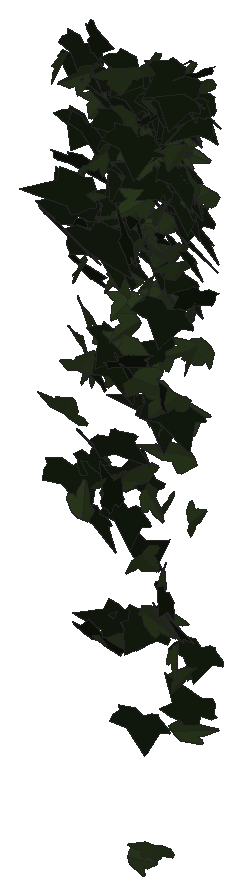
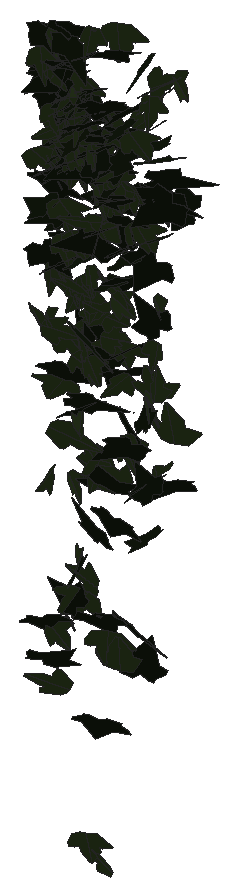
# SketchUp Ruby script. Lengths in millimetres.
U = 1.mm
M = Sketchup.active_model
def pt(a) = Geom::Point3d.new(a.map { |v| v * U })
def face(e, loops, mat)
  f = e.add_face(loops[0].map { |a| pt(a) })
  loops[1..].each { |l| e.add_face(l.map { |a| pt(a) }).erase! }
  f.material = f.back_material = mat if mat
  f
end
# faces: each face lists its corners as indices into pts; further lists are holes
def faces(e, pts, list, mat = nil) = list.each { |f| face(e, (f[0].is_a?(Array) ? f : [f]).map { |l| l.map { |i| pts[i] } }, mat) }
# xy, xz, yz: faces in a plane at the given z, y or x. An outline is a flat list of corners, or four numbers for a rectangle; further outlines are holes
def ring(l) = l.size == 4 ? [[l[0], l[1]], [l[2], l[1]], [l[2], l[3]], [l[0], l[3]]] : l.each_slice(2).to_a
def flat(e, list, mat, &to3) = list.each { |f| face(e, (f[0].is_a?(Array) ? f : [f]).map { |l| ring(l).map { |u, v| to3.(u, v) } }, mat) }
def xy(e, z, list, mat = nil) = flat(e, list, mat) { |x, y| [x, y, z] }
def xz(e, y, list, mat = nil) = flat(e, list, mat) { |x, z| [x, y, z] }
def yz(e, x, list, mat = nil) = flat(e, list, mat) { |y, z| [x, y, z] }
def lines(e, pts, list) = list.each { |a, b| e.add_line(pt(pts[a]), pt(pts[b])) }
# prism: a flat outline (further loops are holes) pulled along v
def prism(e, loops, v, mat = nil)
  f = face(e, loops, mat); d = Geom::Vector3d.new(v.map { |x| x * U })
  f.pushpull(f.normal.samedirection?(d) ? d.length : -d.length)
end
def box(e, o, s, mat = nil) = prism(e, [[o, [o[0] + s[0], o[1], o[2]], [o[0] + s[0], o[1] + s[1], o[2]], [o[0], o[1] + s[1], o[2]]]], [0, 0, s[2]], mat)
def at(x, y, z, deg = 0) = Geom::Transformation.translation(pt([x, y, z])) * Geom::Transformation.rotation(ORIGIN, Z_AXIS, deg.degrees)
def axes(o, x, y, z) = Geom::Transformation.new([*x, 0, *y, 0, *z, 0, *pt(o).to_a, 1])
def part(name) = M.definitions.add(name)
# library, detail: a bought-in or finely detailed component or shape, given as its bounding box
def library(name, o, s) = part(name).tap { |d| box(d.entities, o, s) }
def detail(e, o, s) = box(e.add_group.entities, o, s)
def put(e, d, t, mat = nil) = e.add_instance(d, t).tap { |i| i.material = mat if mat }
def group(e, t, mat = nil) = e.add_group.tap { |g| g.transformation = t; g.material = mat if mat }.entities
root = M.entities
M.materials.add("efeu1").color = [18, 25, 13]
M.materials.add("efeu2").color = [43, 57, 29]
c1 = part("ivyleaf_10")
p = [[0,12.8,-0.8],[-1.5,51.3,-10.9],[-4.9,51,-11.6],[-13.6,26.5,-7.3],[-13.2,15.9,-4.6],[-21.1,19.3,-7.2],
  [-29.5,16.3,-8.3],[-29.2,8.3,-6.2],[-19.7,-9.8,0.5],[-7.6,-13,4],[1,-12.2,5.8],[-0.4,51.1,-11.1],
  [-1.5,51.1,-10.9],[1,-12.4,5.9],[16.9,-12.4,3.5],[35.1,9.1,-5.1],[35,12.9,-6.1],[20.5,16.4,-4.9],
  [15.8,15,-3.8],[15.3,27.6,-7.1],[12.8,31.3,-7.8]]
faces(c1.entities,p,[[0,1,2,3,4,5,6,7,8,9,10],[11,12,0,13,14,15,16,17,18,19,20]],"efeu2")
c2 = part("ivyleaf_9")
p = [[39.1,54.8,31.7],[34.5,51.8,30.2],[-5.3,25.2,17.3],[-17.9,28.3,20.9],[-21.6,21.7,17],[-20.2,4.3,5.3],
  [-22.9,-0.3,2.5],[-17.1,-4,-0.6],[-2,-2.1,-1.2],[-0.7,-15.4,-10.1],[16.6,-22.3,-16.7],[21.1,-15.1,-12.5],
  [32.7,-10.7,-11],[46.1,-1.8,-6.6],[30.8,11.2,3.8]]
faces(c2.entities,p,[[0,1,2,3,4,5,6,7,8,9,10,11,12,13,14]],"efeu1")
put(root,c1,axes([1159.9,911.5,1594.2],[0.32513,-0.7471,0.35],[0.24171,-0.32935,-0.76501],[1.55146,0.20788,0.04584]))
put(root,c1,axes([1156.6,970.6,1037.6],[-1.07605,0.47625,0.41907],[0.55178,-0.30531,0.73812],[1.07388,0.63409,0.04065]))
put(root,c2,axes([1144.9,952.8,1391],[1.62557,0.19363,0.00813],[0.01368,0.00506,-0.87579],[-0.36858,0.85415,0.00335]))
put(root,c1,axes([1164.6,958.1,1198.9],[0.31371,-0.73635,0.01947],[-0.00898,-0.021,-0.75452],[1.40188,0.16464,-0.00919]))
put(root,c1,axes([1169.3,960.4,1115.8],[-0.99769,0.51043,0.28692],[-0.38193,0.20516,-0.73164],[-1.04692,-0.56128,-0.00651]))
put(root,c1,axes([1175.6,969.8,991.9],[0.31863,-0.24231,0.79637],[-0.89433,0.643,0.29443],[-1.30769,-0.49879,-0.00731]))
put(root,c1,axes([1157.6,923.9,940.9],[-1.65035,0.0751,0.31552],[0.57406,-0.14434,0.86332],[0.22691,0.91141,0.11072]))
put(root,c2,axes([1143,984.8,1174.3],[1.23837,-0.18816,-0.40424],[0.76944,-0.05265,0.67526],[-0.35791,-0.76421,0.05301]))
put(root,c2,axes([1165.8,964.2,1278.3],[0.99581,0.56044,0.06902],[0.09755,0.04657,-0.7667],[-1.07026,0.5257,-0.00566]))
put(root,c2,axes([1166.9,994.2,986.3],[-0.32289,-0.14497,0.77042],[-0.11432,-0.78354,-0.16066],[1.48761,-0.09168,0.15487]))
put(root,c2,axes([1159,939.7,1587.2],[0.69414,-0.6805,-0.43662],[-0.30896,0.4076,-0.77087],[1.50744,0.39689,0.04306]))
put(root,c1,axes([1175.9,966,1015.5],[0.64827,-0.72726,-0.00598],[-0.0036,0.00572,-0.80307],[1.38416,0.34063,0.00072]))
put(root,c2,axes([1166.5,960.3,1600.1],[-0.28503,-0.77891,0.2669],[-0.06559,-0.26512,-0.79303],[1.56566,-0.15291,0.01537]))
put(root,c2,axes([1160.8,983,1536.1],[0.378,-0.7746,-0.18675],[-0.07957,0.18207,-0.79965],[1.51437,0.20291,0.0046]))
put(root,c2,axes([1174.5,957.7,1459.9],[-0.82889,-0.61017,0.31763],[0.07587,-0.39769,-0.70932],[1.30699,-0.36388,0.24261]))
put(root,c1,axes([1178,942.1,1377],[0.47899,-0.80206,0.1969],[0.08656,-0.19207,-0.8405],[1.56941,0.25538,-0.01374]))
put(root,c2,axes([1158.5,982.7,860.2],[1.07212,-0.24968,-0.50922],[0.88478,-0.20781,0.61618],[-0.61825,-0.73038,-0.00124]))
put(root,c2,axes([1174.8,975.2,1316.8],[-0.47432,-0.68277,0.30544],[0.08624,-0.33514,-0.71219],[1.42094,-0.20758,0.14519]))
put(root,c1,axes([1186.8,950.5,1562.9],[-0.32026,-0.75005,-0.31521],[0.13106,0.3076,-0.76869],[1.54287,-0.18182,-0.00013]))
put(root,c1,axes([1180.6,940,1021.9],[-1.07087,-0.52934,0.14175],[0.19473,0.09812,0.77253],[-1.0246,0.57189,-0.00134]))
put(root,c2,axes([1175.3,921.5,845.1],[-0.49527,-0.77132,-0.42107],[0.33043,0.38536,-0.81321],[1.6395,-0.31067,0.0367]))
put(root,c1,axes([1196.5,981,1505.4],[-0.74088,-0.61442,0.38107],[-0.16276,-0.39063,-0.71719],[1.36636,-0.37969,0.1212]))
put(root,c2,axes([1187,973.3,511.2],[1.29406,-0.40982,0.23307],[-0.3807,0.11962,0.79389],[-0.81251,-0.70875,-0.00077]))
put(root,c1,axes([1200.1,963.2,1327.8],[-0.69097,-0.7546,0.27247],[-0.20373,-0.25084,-0.83732],[1.51326,-0.37833,0.01169]))
put(root,c2,axes([1214,882,1341.6],[-1.74225,0.11244,-0.06237],[-0.12214,-0.01097,0.92212],[0.21206,0.91749,0.01867]))
put(root,c1,axes([1202.7,917.4,1575.1],[-0.1276,0.01468,-0.90738],[-0.66609,-0.83989,0.01228],[-1.59355,0.34989,0.06753]))
put(root,c2,axes([1223,888.6,1378.2],[-0.9253,-0.21057,0.75866],[-1.34211,-0.28011,-0.52965],[0.66645,-0.85644,-0.0133]))
put(root,c2,axes([1198,940.9,1634],[0.75203,-0.0654,-0.75758],[-1.02703,0.57738,-0.33131],[1.01958,0.62984,0.22505]))
put(root,c2,axes([1185.2,954.1,854.1],[0.41859,-0.74322,-0.33026],[-0.19077,0.31474,-0.77506],[1.53607,0.24162,-0.00626]))
put(root,c2,axes([1183.7,961.5,752.7],[0.43473,-0.79499,0.10746],[0.0864,-0.09874,-0.827],[1.52434,0.23232,0.01623]))
put(root,c2,axes([1188.9,942,1470],[0.00597,-0.7575,0.31667],[0.23096,-0.31277,-0.74936],[1.54541,0.04967,0.11077]))
put(root,c2,axes([1175.9,865,1327.4],[1.2245,-0.64937,0.36279],[0.46055,-0.27085,-0.91396],[1.33867,0.68717,-0.01741]))
put(root,c1,axes([1222.3,976,1402.5],[-1.43367,0.2302,0.10623],[-0.22868,-0.03091,-0.78507],[-0.42489,-0.76012,0.0641]))
put(root,c2,axes([1243.9,949.8,574.4],[-1.01617,0.49004,0.36474],[-0.52043,0.24144,-0.72469],[-1.03964,-0.59985,0.00627]))
put(root,c2,axes([1205.6,978.3,1556.4],[0.44313,-0.66748,-0.43378],[-0.15619,0.42941,-0.70482],[1.50696,0.24079,0.0545]))
put(root,c1,axes([1208.9,979,1398.4],[-0.9936,0.38002,-0.45111],[0.56513,-0.3512,-0.6395],[-0.96997,-0.5939,0.08951]))
put(root,c2,axes([1212,977.4,1237.5],[-0.43904,-0.7832,-0.18856],[0.11826,0.17825,-0.81642],[1.52861,-0.23874,0.00901]))
put(root,c2,axes([1211,984.3,1268.4],[-0.28935,-0.63684,0.42663],[0.16004,-0.44617,-0.63605],[1.45007,-0.07783,0.15533]))
put(root,c1,axes([1226.2,985.1,1194.2],[0.007,-0.66469,0.4371],[-0.03974,-0.43704,-0.66441],[1.51353,-0.0084,-0.01947]))
put(root,c1,axes([1227.7,978.7,515.4],[-1.33004,-0.42344,-0.02594],[-0.03098,-0.02319,0.81704],[-0.8068,0.69894,0.01139]))
put(root,c2,axes([1206.3,985,1461.1],[0.98898,-0.59817,0.07715],[0.2035,-0.00886,-0.78885],[1.12969,0.52526,0.07456]))
put(root,c2,axes([1237.6,993.7,1384.1],[-1.14294,-0.50149,0.0585],[-0.10989,-0.02209,-0.78213],[0.9546,-0.60297,-0.02]))
put(root,c2,axes([1214.8,985.6,1517.1],[0.54786,-0.76354,-0.00955],[0.01553,0.01328,-0.81591],[1.45321,0.28772,0.01232]))
put(root,c1,axes([1237.2,866,812.6],[0.25423,0.69526,-0.59978],[0.06624,0.60182,0.70538],[1.7463,-0.12405,0.06056]))
put(root,c2,axes([1236.4,989.1,1379.2],[-0.89768,-0.59525,0.19565],[-0.03918,-0.23003,-0.74949],[1.19187,-0.45589,0.12272]))
put(root,c1,axes([1229.9,977.3,1423.2],[0.74981,0.68512,-0.08166],[-0.07296,-0.07215,-0.79031],[-1.31111,0.39582,-0.00272]))
put(root,c2,axes([1235.6,955.6,1083.8],[-0.6021,-0.65996,0.4688],[-0.30155,-0.44311,-0.73072],[1.51087,-0.35144,0.04098]))
put(root,c2,axes([1223.6,966.7,1285.3],[0.23928,-0.73854,-0.2323],[-0.01532,0.23409,-0.74857],[1.4734,0.12237,0.02994]))
put(root,c2,axes([1247.5,969.5,1334],[-1.32564,-0.35985,0.00332],[-0.0049,-0.00225,-0.78399],[0.68488,-0.69654,0.00082]))
put(root,c1,axes([1244,977.1,1150.1],[-0.57028,-0.35618,0.60833],[0.09915,-0.67039,-0.36685],[1.33796,-0.10214,0.28647]))
put(root,c2,axes([1225.5,968.1,1295.9],[-0.0614,0.11536,0.80072],[0.507,-0.75515,0.11953],[1.4538,0.26823,-0.00787]))
put(root,c1,axes([1236.8,954.7,1029.5],[-0.27344,-0.49022,-0.63426],[0.73946,0.52103,-0.49072],[1.33447,-0.38917,0.14196]))
put(root,c1,axes([1245.2,960.4,1299.7],[-1.23239,-0.60385,0.04266],[0.07657,0.01941,0.8853],[-1.14956,0.64865,0.01323]))
put(root,c2,axes([1231.7,948,907.8],[0.00567,-0.2647,-0.73262],[0.29126,0.71854,-0.259],[1.45364,-0.14294,0.05475]))
put(root,c1,axes([1252.9,976.6,1112],[-0.12485,-0.34481,0.77559],[0.06473,-0.77835,-0.34315],[1.61411,0.00455,0.07375]))
put(root,c1,axes([1247.2,952.9,1089.6],[1.55003,0.29656,-0.10394],[-0.19078,-0.02849,-0.86671],[-0.56683,0.82054,0.00747]))
put(root,c2,axes([1238.3,954.6,1046],[-0.24453,-0.75221,-0.29134],[0.19676,0.27723,-0.76135],[1.52257,-0.15663,0.0516]))
put(root,c1,axes([1254.8,976.8,552.4],[-1.26054,-0.4927,-0.06058],[0.09168,0.03673,-0.82549],[0.94031,-0.66408,-0.00072]))
put(root,c1,axes([1225.2,973.1,1192],[0.453,-0.3089,-0.7533],[1.09062,-0.49396,0.38362],[-1.10075,-0.61654,0.07008]))
put(root,c2,axes([1240,984.3,1216.9],[-0.29812,-0.63717,0.38782],[0.21479,-0.41196,-0.63125],[1.40328,-0.07231,0.17901]))
put(root,c2,axes([1263.3,954.7,1461.2],[-1.11908,-0.55261,0.41769],[-0.43747,-0.36119,-0.80143],[1.24366,-0.6243,0.09394]))
put(root,c2,axes([1244.6,959.6,1494.2],[-0.56841,-0.70015,-0.37676],[0.24629,0.35429,-0.76097],[1.49302,-0.325,-0.01791]))
put(root,c2,axes([1238.6,975.1,1435.3],[1.29334,-0.38537,-0.15543],[-0.23342,0.09865,-0.78083],[0.7556,0.69009,0.02482]))
put(root,c2,axes([1249.2,968.3,773.2],[-1.10261,-0.14104,-0.55861],[1.04265,0.11038,-0.59604],[0.33945,-0.79719,0.0163]))
put(root,c1,axes([1250.4,949.3,829.9],[-0.29958,-0.68372,0.48925],[0.21864,0.47559,0.70159],[-1.58508,0.19482,0.00431]))
put(root,c2,axes([1264.3,974,1481],[-1.08865,-0.5601,0.03966],[-0.01387,-0.0492,-0.8],[1.06856,-0.57127,0.03002]))
put(root,c1,axes([1266.3,950,1505],[1.07706,-0.46479,-0.38444],[-0.31992,0.38474,-0.7126],[1.10248,0.56571,0.16879]))
put(root,c1,axes([1266.3,980.6,1381],[-0.04993,-0.77131,-0.15454],[-0.02635,0.15505,-0.77153],[1.49691,-0.023,-0.01874]))
put(root,c1,axes([1266.7,888.1,1464.8],[-0.04376,0.06424,-0.93277],[-0.38136,-0.91171,-0.05785],[-1.73811,0.19842,0.03617]))
put(root,c2,axes([1267.1,967.6,825],[-1.2747,-0.08236,0.4732],[0.89173,0.06664,0.67477],[-0.20115,0.81735,-0.00733]))
put(root,c2,axes([1246,985.9,1387.1],[0.75102,-0.68548,0.1194],[0.0933,-0.10953,-0.79086],[1.32097,0.39746,-0.01202]))
put(root,c2,axes([1273.5,967.3,1318.2],[0.40702,-0.05524,-0.82809],[-1.21009,0.53871,-0.20014],[1.01518,0.66428,0.09344]))
put(root,c1,axes([1277.7,900.2,871.4],[-0.26179,-0.93242,0.07887],[-0.02803,-0.07755,-0.94251],[1.7807,-0.1383,-0.00324]))
put(root,c2,axes([1264.7,979.7,1546],[-0.62954,-0.6871,-0.27987],[0.23336,0.25158,-0.76258],[1.3926,-0.35277,0.00127]))
put(root,c2,axes([1282.1,971.8,1295.5],[-0.78481,-0.31937,0.57581],[-0.57321,-0.51268,-0.50005],[1.11438,-0.48863,0.14831]))
put(root,c1,axes([1251.8,985.2,129.5],[0.31487,-0.26715,-0.63044],[0.90923,-0.41959,0.30317],[-0.93352,-0.49877,0.08264]))
put(root,c2,axes([1304.9,966.5,1419],[-0.34518,0.12053,0.79075],[-1.28531,0.41142,-0.21761],[-0.81577,-0.69922,0.00827]))
put(root,c1,axes([1272.8,968.4,1487.6],[1.35718,-0.37726,-0.01934],[-0.03251,0.00907,-0.80675],[0.71822,0.71331,0.00003]))
put(root,c2,axes([1269.5,981.4,394.6],[-0.96803,-0.46562,-0.37996],[0.5389,0.25339,-0.68956],[1.00887,-0.58212,0.00376]))
put(root,c1,axes([1282.6,978.2,1449.8],[-0.11742,-0.78049,-0.21693],[0.00011,0.21756,-0.78275],[1.54174,-0.05946,-0.01647]))
put(root,c2,axes([1263.1,948.7,1047.4],[0.14122,-0.54991,0.6777],[0.13443,-0.67413,-0.55474],[1.65555,0.10165,-0.01276]))
put(root,c1,axes([1284.2,983.9,1057.1],[-0.21478,-0.71523,0.10454],[-0.00319,-0.10555,-0.72393],[1.37569,-0.11191,0.01464]))
put(root,c2,axes([1274.9,979.1,1456.8],[-0.45566,-0.77666,0.02771],[-0.01084,-0.02724,-0.81272],[1.47904,-0.23947,0.00258]))
put(root,c2,axes([1262.9,862.2,1333.2],[-0.19609,-0.62569,-0.77186],[0.43463,0.74031,-0.6306],[1.84041,-0.2415,0.06668]))
put(root,c1,axes([1272.5,971.1,1152.4],[0.54648,0.40063,-0.56727],[0.56471,0.48422,0.49217],[1.19501,-0.41203,0.02683]))
put(root,c2,axes([1287.8,972,579.5],[-1.28504,-0.49233,-0.06076],[0.09264,0.03638,-0.83563],[0.93956,-0.67695,-0.00072]))
put(root,c1,axes([1281.7,967.1,857.2],[-0.59925,-0.69452,-0.3284],[0.30933,0.28665,-0.76208],[1.42904,-0.35329,0.02725]))
put(root,c2,axes([1272.2,921,1075.5],[0.96238,0.51382,0.36711],[0.48918,0.26212,-0.72091],[-1.09779,0.56724,0.00059]))
put(root,c2,axes([1261.8,994,1431.9],[0.23986,-0.47042,0.6314],[0.49978,-0.57772,-0.48284],[1.41274,0.28425,0.06361]))
put(root,c2,axes([1284.3,973.2,1406],[-1.20748,-0.40163,-0.27007],[0.5004,0.08782,-0.74828],[0.77335,-0.68392,0.06251]))
put(root,c2,axes([1292.3,937.9,1613],[-1.04686,-0.61416,0.19272],[-0.13741,-0.19304,-0.82123],[1.21734,-0.54994,0.07304]))
put(root,c1,axes([1290.2,979.3,1175.7],[-0.32461,-0.75449,-0.19553],[0.11251,0.18706,-0.77336],[1.47911,-0.17981,0.01591]))
put(root,c1,axes([1296,980.2,164.5],[-1.13209,-0.38718,0.09762],[-0.15521,-0.05366,-0.70974],[0.74393,-0.6004,0.00048]))
put(root,c2,axes([1316.4,980.9,977.3],[-0.55295,-0.36184,-0.62774],[-0.79595,-0.46854,0.46363],[-1.12607,0.50886,-0.01947]))
put(root,c2,axes([1263.8,971.8,1284.7],[1.36129,0.08674,0.40551],[0.76742,0.04329,-0.72049],[-0.18428,0.82108,-0.00486]))
put(root,c1,axes([1297.3,967.9,1214.8],[0.06087,-0.74517,-0.15737],[0.06568,0.15876,-0.74476],[1.44799,0.02412,0.0404]))
put(root,c1,axes([1298.5,943.5,1293],[-0.02154,-0.77015,0.09847],[0.03764,-0.09873,-0.76995],[1.47721,-0.00872,0.02105]))
put(root,c1,axes([1302,889.4,1628.6],[-1.03923,-0.76578,-0.05381],[0.0725,0.03892,-0.94048],[1.45922,-0.54731,0.00841]))
put(root,c2,axes([1315.4,849.8,864.8],[-0.08495,0.21702,0.92704],[-0.214,0.92036,-0.22087],[-1.79936,-0.11971,-0.0175]))
put(root,c1,axes([1297.3,972.8,1436.9],[-1.04801,0.57233,-0.01593],[0.02228,-0.01085,-0.79422],[-1.08946,-0.55078,-0.00091]))
put(root,c1,axes([1309.1,931,1377],[-0.53974,-0.31519,0.76725],[-0.14838,-0.79714,-0.35629],[1.57166,-0.1835,0.22986]))
put(root,c2,axes([1325.4,964.7,1093.1],[-0.82137,0.66601,0.29854],[-0.30552,0.25171,-0.79361],[-1.35506,-0.46045,-0.00203]))
put(root,c1,axes([1296.2,941.3,1454.6],[1.24289,0.4741,-0.03684],[-0.05664,-0.02171,-0.807],[-0.90325,0.65373,-0.00008]))
put(root,c2,axes([1319.8,951.6,1410.8],[-1.47908,-0.42242,0.22217],[-0.36457,-0.11279,-0.88451],[0.832,-0.80038,0.00739]))
put(root,c1,axes([1278.9,967.8,1312],[0.28923,-0.12017,-0.83466],[1.41984,0.41455,0.07615],[0.74821,-0.74021,0.17815]))
put(root,c1,axes([1307.3,980.8,1084.2],[0.63547,-0.61222,-0.24156],[-0.01631,0.2668,-0.68804],[1.25249,0.31409,0.1136]))
put(root,c1,axes([1310.5,988.4,1438.7],[-0.34856,-0.71078,0.31527],[0.03585,-0.32786,-0.72822],[1.47943,-0.15952,0.09193]))
put(root,c1,axes([1282.3,965.9,1287.5],[-0.0735,0.06399,-0.86395],[1.07194,-0.65523,-0.07371],[-1.25275,-0.56442,-0.01238]))
put(root,c1,axes([1310.4,977.8,1445.6],[0.0482,-0.8054,0.11298],[0.01119,-0.11285,-0.80579],[1.5478,0.0259,0.00231]))
put(root,c1,axes([1307.3,992.4,1061.9],[-0.37874,-0.48349,0.53658],[0.22847,-0.57097,-0.46996],[1.35551,-0.03885,0.22913]))
put(root,c2,axes([1296.9,989.3,1500.7],[-0.22216,-0.78873,-0.13775],[0.1348,0.12848,-0.79572],[1.51785,-0.12685,0.05051]))
put(root,c2,axes([1300.4,989.3,1241.9],[-0.20662,-0.6919,0.29457],[0.05837,-0.30145,-0.69676],[1.43001,-0.08767,0.071]))
put(root,c1,axes([1314.3,969.4,1191.1],[-0.44757,-0.55927,0.45625],[0.09429,-0.49123,-0.57662],[1.37043,-0.14886,0.18868]))
put(root,c1,axes([1306,987.4,929.5],[-0.05808,-0.34319,-0.65587],[0.05666,-0.65646,0.34212],[-1.40767,-0.01226,0.04083]))
put(root,c2,axes([1297.3,948.6,712],[-0.44093,0.46867,0.64282],[0.52855,-0.57975,0.52278],[1.4188,0.36163,0.00502]))
put(root,c2,axes([1307.4,920.9,1496.2],[-0.73521,-0.80004,-0.10881],[0.06761,0.10366,-0.88833],[1.53517,-0.38771,-0.01299]))
put(root,c2,axes([1329.8,943.1,1538.1],[-0.69022,0.72173,-0.17639],[0.0544,-0.18258,-0.80584],[-1.41297,-0.35958,0.05514]))
put(root,c1,axes([1318,953.3,1041.7],[-0.03989,-0.82382,-0.06096],[0.01408,0.06079,-0.82407],[1.57212,-0.02145,0.00583]))
put(root,c1,axes([1319,969,1466],[-0.07385,-0.78761,-0.13662],[0.06772,0.13494,-0.78805],[1.51985,-0.04428,0.02848]))
put(root,c2,axes([1307.9,984.1,964.5],[-0.30045,-0.84297,0.08874],[-0.02898,-0.08743,-0.85762],[1.61295,-0.1586,0.00112]))
put(root,c1,axes([1324.2,975,1274],[-0.69287,-0.64306,0.23922],[-0.10983,-0.24115,-0.73608],[1.30119,-0.36278,0.06525]))
put(root,c1,axes([1321.7,968.8,1534.2],[0.48552,-0.36488,0.71621],[-0.54009,0.66215,0.43841],[-1.43128,-0.37363,0.07752]))
put(root,c2,axes([1309.4,994.1,1432.4],[-0.23543,-0.76671,0.15449],[-0.06169,-0.15125,-0.77658],[1.48724,-0.12764,-0.00776]))
put(root,c1,axes([1314.9,980.4,677.3],[-0.01859,0.06863,-0.73588],[0.04315,-0.73557,-0.0689],[-1.40595,-0.02348,0.00762]))
put(root,c1,axes([1323.7,979.8,1523.4],[-0.76998,-0.7041,-0.01924],[0.12983,-0.01708,-0.80924],[1.33425,-0.40467,0.06764]))
put(root,c2,axes([1314.9,982.2,1504.6],[-0.52554,-0.73945,0.17309],[0.08186,-0.19911,-0.78199],[1.44304,-0.258,0.1074]))
put(root,c1,axes([1319.9,967,1171.5],[-0.55749,-0.52283,-0.46955],[0.38692,0.42391,-0.59883],[1.28025,-0.35578,-0.02349]))
put(root,c1,axes([1351.9,979.1,905.2],[0.46313,0.0442,-0.83711],[-1.58621,0.10625,-0.23667],[0.17111,0.86527,0.07182]))
put(root,c1,axes([1314.4,968.8,605.1],[-1.47846,0.00632,-0.33487],[0.63743,0.01008,-0.77676],[-0.00346,-0.84587,-0.01176]))
put(root,c2,axes([1309,984.5,1499],[0.24564,-0.7895,0.08995],[0.022,-0.08925,-0.79998],[1.51214,0.12955,-0.00298]))
put(root,c1,axes([1324.5,932.1,1635.2],[-0.30456,-0.728,-0.40796],[0.22682,0.3912,-0.74484],[1.57197,-0.19749,0.02843]))
put(root,c2,axes([1304.4,977.3,1419.7],[1.49879,-0.11105,0.00831],[0.01641,0.00166,-0.79529],[0.2113,0.78755,0.00285]))
put(root,c2,axes([1308.7,991,1489.3],[0.33691,-0.78367,0.04469],[0.01028,-0.04459,-0.8034],[1.49387,0.17704,-0.00455]))
put(root,c1,axes([1300,990.6,1184.1],[-0.27072,-0.07055,-0.7736],[1.23711,-0.44144,-0.07926],[-0.80952,-0.65102,0.13758]))
put(root,c2,axes([1323.5,972.1,1542.4],[-0.58414,-0.75596,0.13747],[-0.01765,-0.14438,-0.81464],[1.46223,-0.30374,0.04508]))
put(root,c2,axes([1308.4,987.1,1461.8],[0.60317,-0.79261,0.11744],[0.04453,-0.11709,-0.85335],[1.52431,0.31706,-0.02154]))
put(root,c1,axes([1329.1,968.7,1409.2],[-0.42886,-0.71646,-0.31183],[0.20453,0.29304,-0.75094],[1.47299,-0.24929,0.01348]))
put(root,c1,axes([1341.4,985.4,1332.4],[-1.04222,-0.42487,0.36354],[-0.38918,-0.32143,-0.68368],[0.99051,-0.57335,0.11389]))
put(root,c1,axes([1332.3,971.8,819.3],[0.23209,-0.76393,0.0114],[-0.00462,-0.01193,-0.77359],[1.45406,0.1219,-0.00428]))
put(root,c1,axes([1340.5,945.5,1546.4],[-1.54408,-0.01771,0.15561],[-0.29656,0.00872,-0.81141],[0.02997,-0.82605,-0.0119]))
put(root,c1,axes([1344.1,972.2,1568.3],[-1.53536,-0.03071,0.18719],[-0.35596,-0.00769,-0.80731],[0.06024,-0.82812,0.00056]))
put(root,c1,axes([1338,974.6,1512.9],[-0.60883,0.68504,0.29117],[-0.38016,0.22629,-0.75186],[-1.3647,-0.36866,0.07954]))
put(root,c2,axes([1314.2,981,1540.2],[0.98377,-0.63502,-0.09522],[0.0172,0.12942,-0.81405],[1.22197,0.50942,0.08812]))
put(root,c2,axes([1319,984.4,1516.4],[-0.00482,-0.63401,0.51191],[0.30212,-0.50249,-0.62156],[1.52116,0.09779,0.12507]))
put(root,c1,axes([1314.7,983.5,1175.7],[-0.38415,0.06171,0.76413],[1.26232,-0.38217,0.20607],[0.73162,0.69179,0.04568]))
put(root,c2,axes([1319.3,982.4,1513.5],[0.41658,-0.77694,0.1094],[0.04823,-0.10651,-0.80717],[1.49248,0.2203,-0.00445]))
put(root,c2,axes([1350.8,956.7,1621.4],[-0.13676,0.84748,-0.06127],[-0.00731,-0.06181,-0.85047],[-1.61711,-0.07139,0.00902]))
put(root,c1,axes([1312.9,941,834.9],[0.50577,-0.1273,0.81893],[1.32083,-0.4359,-0.29297],[0.86216,0.74247,-0.03159]))
put(root,c2,axes([1324.8,970.1,645.8],[0.46005,-0.33736,-0.74303],[1.01439,-0.52154,0.41019],[-1.17603,-0.58183,0.06315]))
put(root,c2,axes([1326.8,982.3,1521.9],[0.10968,-0.81127,-0.0914],[0.02728,0.09262,-0.81305],[1.55354,0.05565,0.02073]))
put(root,c2,axes([1344.4,964.2,1547.7],[-0.41289,-0.36537,0.7381],[0.72787,0.6313,0.42491],[-1.38819,0.43968,0.00326]))
put(root,c2,axes([1353.5,843.8,1335.6],[-0.23118,-0.53915,0.79492],[0.28649,0.78066,0.55249],[-1.80545,0.19291,-0.01411]))
put(root,c2,axes([1329.4,960.9,1598.4],[0.0426,-0.83273,-0.14823],[0.03572,0.14874,-0.83273],[1.60936,0.01874,0.02241]))
put(root,c2,axes([1320.9,978.1,591.3],[0.32699,-0.35272,0.70217],[0.56019,-0.63754,-0.39228],[1.38663,0.34074,-0.00711]))
put(root,c1,axes([1351.1,970.2,1256.6],[-0.54885,-0.76413,-0.00461],[0.00097,0.00474,-0.81674],[1.45432,-0.28838,-0.0012]))
put(root,c2,axes([1346.7,973.9,1526.7],[-0.57831,-0.56755,0.50605],[-0.30451,-0.48503,-0.64006],[1.41478,-0.33639,0.06909]))
put(root,c1,axes([1318.9,936.5,614],[-0.07761,-0.01524,0.83192],[1.51109,-0.24982,0.03434],[0.47361,0.79457,0.02675]))
put(root,c1,axes([1351.6,931.3,1379.7],[-0.01243,-0.79512,0.00393],[0.00026,-0.00393,-0.79515],[1.51329,-0.00653,0.00017]))
put(root,c1,axes([1335.1,963.3,1470.3],[-0.9184,-0.46285,-0.4604],[0.90399,0.14385,-0.64246],[0.85238,-0.65125,0.1853]))
put(root,c1,axes([1362,990.5,1098.4],[-0.18837,-0.2883,0.69705],[-0.48549,-0.64882,-0.30457],[1.35104,-0.27334,-0.01226]))
put(root,c2,axes([1333,987.2,1535.8],[0.32816,-0.77271,-0.18191],[0.07542,0.1943,-0.78777],[1.50894,0.15834,0.07894]))
put(root,c2,axes([1331.5,972.3,1416.8],[0.7738,-0.68072,-0.04764],[-0.03273,0.04522,-0.79285],[1.2983,0.40686,0.00841]))
put(root,c2,axes([1364.7,953.5,1499.7],[-0.478,0.66674,-0.46076],[0.31429,-0.43016,-0.71247],[-1.5101,-0.30057,-0.00244]))
put(root,c1,axes([1375.5,967.3,1424.9],[-0.93972,0.3392,0.53412],[-1.05235,0.09802,-0.5734],[-0.58537,-0.72074,0.17339]))
put(root,c1,axes([1340.7,885.8,1080.9],[-0.65702,-0.48241,-0.78392],[1.02667,0.57236,-0.58977],[1.41945,-0.63727,0.06372]))
put(root,c1,axes([1361.5,982,1502.6],[-0.69407,-0.72316,0.06062],[0.02625,-0.07474,-0.80861],[1.38089,-0.36206,0.04584]))
put(root,c2,axes([1340.4,954,1553.8],[0.69209,-0.69626,-0.36319],[-0.13477,0.36954,-0.77933],[1.48848,0.35719,0.09831]))
put(root,c2,axes([1343.4,980.5,1224.5],[0.30222,-0.71028,-0.24214],[0.01459,0.24903,-0.72545],[1.42813,0.14776,0.05865]))
put(root,c2,axes([1344.8,919.3,1045.4],[-0.17783,0.11907,0.88174],[0.19392,-0.87932,0.12954],[1.68221,0.11395,0.07827]))
put(root,c1,axes([1366.5,956.6,1301.3],[-0.28411,-0.76224,0.08694],[-0.04214,-0.08425,-0.7767],[1.45948,-0.15081,-0.0055]))
put(root,c2,axes([1375.8,968.1,1523.7],[-0.22424,0.44846,-0.6909],[0.0209,-0.69702,-0.4543],[-1.56751,-0.07344,0.09278]))
put(root,c2,axes([1347.8,973.3,1595.7],[0.2558,-0.8279,-0.0504],[0.00375,0.05138,-0.83868],[1.57857,0.13403,0.01016]))
put(root,c2,axes([1354.6,991.6,1401.5],[-0.14022,-0.77956,0.11326],[0.02463,-0.11494,-0.78268],[1.49903,-0.07103,0.02346]))
put(root,c1,axes([1372.3,949.9,1486],[-0.58885,-0.71411,0.24873],[-0.03805,-0.26093,-0.774],[1.43868,-0.29919,0.08134]))
put(root,c2,axes([1355.8,949.1,1007],[-0.80132,-0.5625,-0.56083],[0.60869,0.46097,-0.70245],[1.38379,-0.5285,-0.01578]))
put(root,c1,axes([1382.2,920.3,1044.8],[-0.92741,-0.59548,0.47357],[-0.45641,-0.4135,-0.7667],[1.37421,-0.5392,0.06496]))
put(root,c1,axes([1353.9,973.5,992.8],[1.22868,0.37467,0.26315],[0.41689,0.14669,-0.74626],[-0.76518,0.68155,0.01596]))
put(root,c1,axes([1353.3,971.6,1470.1],[-0.3678,-0.42858,-0.65534],[0.99966,0.42966,-0.43588],[1.10526,-0.53123,0.17616]))
put(root,c2,axes([1348,979.8,1567.3],[1.4802,-0.2613,-0.01266],[-0.03518,-0.01528,-0.82021],[0.49664,0.7777,-0.02037]))
put(root,c1,axes([1354.5,957.2,556.1],[0.64887,-0.41324,0.65956],[0.81656,-0.501,-0.53567],[1.23591,0.54796,0.00764]))
put(root,c1,axes([1376.3,964.6,522.1],[-0.19667,-0.73527,0.34378],[-0.0796,-0.34127,-0.74248],[1.54271,-0.11135,0.00552]))
put(root,c1,axes([1370.7,972.8,1390.7],[1.01668,-0.60721,-0.00793],[-0.00733,0.00718,-0.80875],[1.15572,0.53421,0.00185]))
put(root,c2,axes([1357.4,969.1,1379.8],[0.26224,-0.76262,-0.13542],[-0.05859,0.13205,-0.77494],[1.47296,0.14103,-0.00672]))
put(root,c1,axes([1376.3,965.7,1560.4],[-0.4016,-0.79134,0.03752],[-0.01414,-0.03685,-0.81898],[1.5077,-0.21113,0.00231]))
put(root,c1,axes([1358,986.7,1566.4],[1.20096,-0.41173,0.31313],[0.62062,-0.06679,-0.74496],[0.76422,0.70127,0.11289]))
put(root,c2,axes([1361.2,960.3,1438.3],[-0.14573,-0.77873,-0.14922],[0.02824,0.14848,-0.78249],[1.50879,-0.078,0.00023]))
put(root,c2,axes([1355.6,965.6,1420.3],[0.52106,-0.76195,-0.06968],[-0.03313,0.06779,-0.80962],[1.45583,0.27426,0.00652]))
put(root,c2,axes([1352.1,972.8,1315.5],[1.25698,-0.52357,-0.07973],[-0.1101,0.05537,-0.84277],[1.00191,0.66294,0.00742]))
put(root,c2,axes([1382.4,977.2,1580.1],[-1.3844,-0.39521,-0.04714],[0.08356,0.01794,-0.82782],[0.75286,-0.72871,0.00519]))
put(root,c2,axes([1388.8,936.8,1630.2],[-1.38826,-0.37271,0.19206],[-0.2834,-0.12998,-0.81781],[0.74596,-0.74301,0.04673]))
put(root,c2,axes([1366.6,970.1,1386.3],[-0.30966,-0.76618,0.0221],[-0.0074,-0.02177,-0.78326],[1.45878,-0.16275,0.00072]))
put(root,c1,axes([1376.1,972.3,1623.5],[0.47574,-0.78312,0.17845],[0.04897,-0.17899,-0.82153],[1.52786,0.24958,-0.02924]))
put(root,c2,axes([1373.7,976.7,1365.1],[-1.27191,-0.22136,-0.39399],[0.70534,0.13405,-0.70395],[0.49221,-0.76412,-0.00936]))
put(root,c2,axes([1354.3,969,1293.6],[0.42992,-0.66532,0.34],[0.29134,-0.30646,-0.70138],[1.39184,0.26966,0.04179]))
put(root,c2,axes([1374,938.5,1593.1],[-0.75556,-0.73355,-0.0254],[0.01992,0.02322,-0.83408],[1.39679,-0.39713,-0.00184]))
put(root,c2,axes([1380,964.3,1575],[-1.05531,-0.59776,0.11302],[-0.00198,-0.15199,-0.80898],[1.15782,-0.5451,0.10163]))
put(root,c1,axes([1384.9,952.9,1526.2],[0.0509,0.33963,-0.7723],[-0.60228,-0.71223,-0.32418],[-1.48845,0.29981,0.10476]))
put(root,c2,axes([1398.8,961.5,454.6],[-1.36918,-0.3952,0.04042],[0.10022,-0.012,0.82003],[-0.74939,0.72044,0.03582]))
put(root,c1,axes([1382.5,964,1187.6],[-0.12513,-0.66927,-0.36742],[0.06469,0.36585,-0.67249],[1.45164,-0.07399,-0.0017]))
put(root,c2,axes([1378.5,992.8,553.6],[-0.73167,-0.65055,-0.08061],[0.07057,0.07173,-0.75564],[1.2456,-0.3862,-0.00455]))
put(root,c1,axes([1378.9,972.7,1105.1],[0.29953,-0.66374,0.32256],[0.27155,-0.29622,-0.67916],[1.378,0.20265,0.06372]))
put(root,c2,axes([1397.1,956.1,1630],[-0.14099,0.79468,-0.33772],[0.05427,-0.33652,-0.79812],[-1.64244,-0.07934,0.00262]))
put(root,c1,axes([1383.7,962.6,804.6],[0.12708,-0.15338,-0.86122],[0.26599,0.8545,-0.14135],[1.64348,-0.12643,0.08947]))
put(root,c2,axes([1396.5,953.5,1553.9],[-1.43186,-0.42413,0.04435],[-0.07397,-0.02137,-0.86366],[0.80823,-0.75335,-0.00047]))
put(root,c1,axes([1384,840.3,790.9],[-0.45563,-0.73155,-0.59799],[0.43014,0.55464,-0.769],[1.74605,-0.32753,0.0334]))
put(root,c1,axes([1389.9,979.8,1596.1],[-0.65428,-0.751,-0.03214],[0.12378,0.00549,-0.82399],[1.42525,-0.34523,0.05681]))
put(root,c2,axes([1386.2,899,1216.7],[-1.2944,-0.34453,-0.35706],[0.59685,0.17101,-0.76234],[0.7318,-0.74887,-0.00982]))
put(root,c1,axes([1401,976.3,1402.4],[-0.83655,-0.40842,0.52634],[-0.44246,-0.49691,-0.57973],[1.18825,-0.47257,0.15469]))
put(root,c2,axes([1372.9,963.4,1559.8],[-0.09581,-0.56971,-0.63941],[0.18321,0.63269,-0.5713],[1.61957,-0.10528,0.0268]))
put(root,c1,axes([1369.8,957.6,414],[-0.32774,-0.2198,0.69867],[0.80593,0.55573,0.27921],[-1.13736,0.45712,-0.00348]))
put(root,c2,axes([1397.9,964.3,1224.9],[0.03748,0.42636,-0.64028],[0.01547,-0.64057,-0.4263],[-1.46396,0.00415,-0.0209]))
put(root,c2,axes([1369.3,993,1321.5],[0.38024,-0.68286,0.34135],[0.27968,-0.31185,-0.70986],[1.42579,0.24328,0.04821]))
put(root,c1,axes([1397,983.5,1112.7],[0.99952,-0.53151,-0.21282],[-0.26633,0.16087,-0.74709],[1.05659,0.54335,0.01301]))
